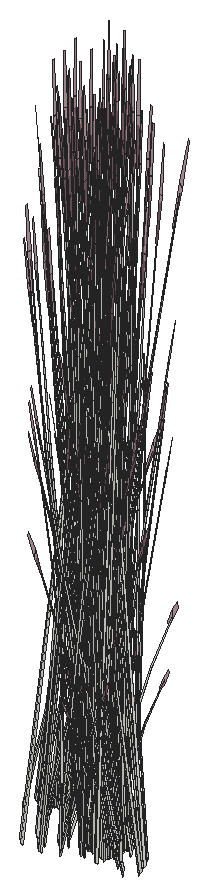
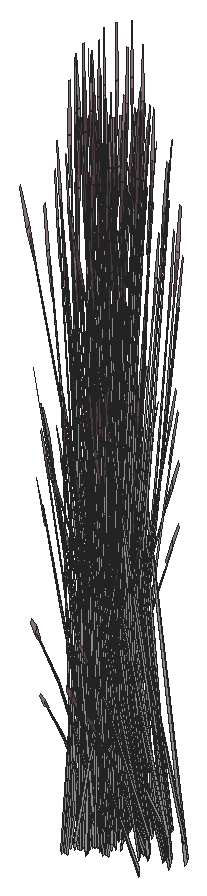
# SketchUp Ruby script. Lengths in inches.
U = 1.inch
M = Sketchup.active_model
def pt(a) = Geom::Point3d.new(a.map { |v| v * U })
def face(e, loops, mat)
  f = e.add_face(loops[0].map { |a| pt(a) })
  loops[1..].each { |l| e.add_face(l.map { |a| pt(a) }).erase! }
  f.material = f.back_material = mat if mat
  f
end
# faces: each face lists its corners as indices into pts; further lists are holes
def faces(e, pts, list, mat = nil) = list.each { |f| face(e, (f[0].is_a?(Array) ? f : [f]).map { |l| l.map { |i| pts[i] } }, mat) }
# xy, xz, yz: faces in a plane at the given z, y or x. An outline is a flat list of corners, or four numbers for a rectangle; further outlines are holes
def ring(l) = l.size == 4 ? [[l[0], l[1]], [l[2], l[1]], [l[2], l[3]], [l[0], l[3]]] : l.each_slice(2).to_a
def flat(e, list, mat, &to3) = list.each { |f| face(e, (f[0].is_a?(Array) ? f : [f]).map { |l| ring(l).map { |u, v| to3.(u, v) } }, mat) }
def xy(e, z, list, mat = nil) = flat(e, list, mat) { |x, y| [x, y, z] }
def xz(e, y, list, mat = nil) = flat(e, list, mat) { |x, z| [x, y, z] }
def yz(e, x, list, mat = nil) = flat(e, list, mat) { |y, z| [x, y, z] }
def lines(e, pts, list) = list.each { |a, b| e.add_line(pt(pts[a]), pt(pts[b])) }
# prism: a flat outline (further loops are holes) pulled along v
def prism(e, loops, v, mat = nil)
  f = face(e, loops, mat); d = Geom::Vector3d.new(v.map { |x| x * U })
  f.pushpull(f.normal.samedirection?(d) ? d.length : -d.length)
end
def box(e, o, s, mat = nil) = prism(e, [[o, [o[0] + s[0], o[1], o[2]], [o[0] + s[0], o[1] + s[1], o[2]], [o[0], o[1] + s[1], o[2]]]], [0, 0, s[2]], mat)
def at(x, y, z, deg = 0) = Geom::Transformation.translation(pt([x, y, z])) * Geom::Transformation.rotation(ORIGIN, Z_AXIS, deg.degrees)
def axes(o, x, y, z) = Geom::Transformation.new([*x, 0, *y, 0, *z, 0, *pt(o).to_a, 1])
def part(name) = M.definitions.add(name)
# library, detail: a bought-in or finely detailed component or shape, given as its bounding box
def library(name, o, s) = part(name).tap { |d| box(d.entities, o, s) }
def detail(e, o, s) = box(e.add_group.entities, o, s)
def put(e, d, t, mat = nil) = e.add_instance(d, t).tap { |i| i.material = mat if mat }
def group(e, t, mat = nil) = e.add_group.tap { |g| g.transformation = t; g.material = mat if mat }.entities
root = M.entities
M.materials.add("LightPink_Translucent").color = [144, 107, 117]
M.materials["LightPink_Translucent"].alpha = 0.75
c1 = part("blade")
p = [[2.15,0.21,22],[0,0.17,0],[0.09,0.45,0],[2.18,0.31,22],[2.29,0.31,22],[0.38,0.45,0],
  [2.48,0.24,33],[2.49,0.24,33],[2.48,0.22,33]]
faces(c1.entities,p,[[0,1,2,3],[4,5,2,3],[6,3,4,7],[8,0,3,6]])
c2 = part("seeds")
p = [[0.3,-0.1,1.38],[-0.01,-0.03,1.59],[-0.01,-0.03,0.03],[0.14,-0.07,-0.07],[0.29,-0.03,3],[0.15,0.01,3.11]]
faces(c2.entities,p,[[0,1,2,3],[1,0,4,5]],"LightPink_Translucent")
c3 = part("blade with seeds")
put(c3.entities,c1,at(0,0,0))
put(c3.entities,c2,axes([2.4,0.25,30.99],[1.5799,-0.05474,1.17369],[-0.12525,1.92788,0.29478],[-0.07173,-0.02425,1.56792]))
put(root,c3,axes([348.41,652.44,624.42],[-0.08753,-0.42921,0.48003],[0.34336,-0.07449,0.3958],[-0.1012,0.10094,0.9933]))
put(root,c3,axes([344.4,651.66,624.44],[-0.09971,0.42522,0.48003],[-0.32782,-0.1454,0.3958],[0.12892,-0.02555,0.9933]))
put(root,c3,axes([348.7,652.1,622.89],[-0.35635,0.30962,-0.29095],[-0.23697,-0.43749,-0.50002],[-0.08792,-0.04443,1.59708]))
put(root,c3,axes([347.72,653.07,624.96],[-0.25132,-0.3182,0.48003],[0.2669,-0.27442,0.3958],[-0.04636,0.14929,0.9933]))
put(root,c3,axes([348.34,652.36,624.42],[-0.2423,-0.19613,0.0643],[0.14107,-0.2793,0.50621],[-0.07768,0.0903,0.77189]))
put(root,c3,axes([345.14,652.99,624.78],[-0.05451,-0.37564,0.35414],[0.31161,-0.09919,-0.4572],[0.0837,0.10765,0.87481]))
put(root,c3,axes([347.9,652.75,622.25],[-0.08291,-0.40636,-0.30978],[0.32928,-0.11539,0.30978],[-0.06638,-0.04686,1.38974]))
put(root,c3,axes([347.625,653.04,624.96],[-0.29004,-0.02173,0.0643],[0.00795,-0.32812,0.50621],[-0.03035,0.12569,0.77189]))
put(root,c3,axes([345.21,651.02,621.9375],[0.21202,0.39143,-0.44739],[-0.32115,0.27564,0.21531],[0.06861,0.04843,1.43643]))
put(root,c3,axes([345.35,650.82,624.2],[-0.30498,-0.24231,1.38283],[0.32203,-0.37727,0.59665],[0.0984,0.22736,1.33663]))
put(root,c3,axes([344.19,652.38,624.42],[0.07571,-0.00789,1.74944],[0.20767,-0.36231,-0.27667],[0.13467,0.04783,0.14031]))
put(root,c3,axes([344.84,653.51,624.43],[0.00104,-0.05646,1.77383],[0.30246,-0.2491,-0.16761],[0.10506,0.08891,0.31391]))
put(root,c3,axes([348.9375,652.43,622.28],[-0.23773,0.35053,-0.62353],[-0.29532,-0.31785,-0.16365],[-0.09526,0.08744,1.37633]))
put(root,c3,axes([345.8125,652.8,622.49],[-0.19872,-0.13409,1.1486],[0.2566,-0.13625,0.84392],[0.06921,0.11541,0.25299]))
put(root,c3,axes([348.57,651.39,624.74],[0.29332,0.1301,0.35414],[-0.08555,0.37955,-0.4572],[-0.11809,0.0348,0.87481]))
put(root,c3,axes([345.09,651.7,622.47],[-0.21807,0.07699,1.1486],[0.10265,-0.31819,0.84392],[0.11568,0.02177,0.25299]))
put(root,c3,axes([348.625,652.57,624.37],[0.09067,0.42583,-0.51099],[-0.34336,0.07449,-0.3958],[-0.0984,0.11438,0.97773]))
put(root,c3,axes([349.48,652.26,621.75],[-0.36714,-0.07646,-0.62353],[0.07747,-0.47163,-0.16365],[-0.10956,-0.05715,1.37633]))
put(root,c3,axes([349.1,652.24,622.69],[-0.34464,-0.37536,-0.25192],[0.29,-0.42149,0.5513],[-0.0928,0.04391,1.68216]))
put(root,c3,axes([348.48,651.875,622.4375],[-0.21202,-0.39143,-0.44739],[0.32115,-0.27564,0.21531],[-0.06861,-0.04843,1.43643]))
put(root,c3,axes([344.47,651.62,624.23],[0.29332,0.1301,-0.35414],[-0.08555,0.37955,0.4572],[0.11809,-0.0348,0.87481]))
put(root,c3,axes([348.9,650.57,624.74],[0.20082,0.29199,0.35414],[-0.2293,0.2764,-0.4572],[-0.1165,-0.04206,0.87481]))
put(root,c3,axes([345.79,650.15,621.75],[0.08291,0.40636,-0.30978],[-0.32928,0.11539,0.30978],[0.06638,0.04686,1.38974]))
put(root,c3,axes([346.41,651.48,622.1],[0.44133,0,0],[0,0.52122,-0.51607],[0,0.11871,1.63711]))
put(root,c3,axes([343.9,652.4375,624.6875],[0.35281,0.01123,-0.71045],[-0.0237,0.47284,0.08574],[0.14947,0.0499,1.00501]))
put(root,c3,axes([348.93,652.16,622.4375],[-0.38326,0.02879,-0.44739],[-0.03466,-0.47788,0.21531],[-0.06861,0.04843,1.43643]))
put(root,c3,axes([344.98,650.8,622.39],[0.35635,-0.30962,-0.29095],[0.23697,0.43749,-0.50002],[0.08792,0.04443,1.59708]))
put(root,c3,axes([344.62,651.54,621.69],[-0.22732,0.05597,1.41583],[-0.03618,-0.44548,0.08104],[0.15921,-0.06743,0.80566]))
put(root,c3,axes([345.84,653.41,622.39],[-0.22633,-0.01463,1.0506],[0.14947,-0.31064,0.58006],[0.08941,0.11036,0.8241]))
put(root,c3,axes([349,653.16,621.71],[-0.33032,-0.23318,-0.49651],[0.19744,-0.41812,0],[-0.07523,-0.05311,1.57504]))
put(root,c3,axes([344.87,651.25,621.2],[-0.01845,-0.0708,1.76342],[0.12793,-0.41416,-0.26939],[0.12905,-0.00596,0.30037]))
put(root,c3,axes([348.46,652.26,624.73],[0.32648,0.25715,-0.1216],[-0.18809,0.3724,-0.67495],[-0.09224,0.12945,1.02557]))
put(root,c3,axes([344.99,653.04,624.42],[-0.03191,-0.04083,1.77383],[0.06981,-0.43764,-0.16761],[0.12571,-0.02796,0.31391]))
put(root,c3,axes([343.67,651.15,623.58],[-0.14639,0.01056,1.71376],[0.09712,-0.45778,0.13857],[0.20862,0.02831,0.73262]))
put(root,c3,axes([348.2,652.96,622.7],[0.33032,0.23318,0.49651],[-0.19744,0.41812,0],[-0.07523,-0.05311,1.57504]))
put(root,c3,axes([349.2,653.4375,622.0625],[-0.22066,0.46731,0],[-0.36918,-0.26061,-0.51607],[-0.08408,-0.05936,1.63711]))
put(root,c3,axes([345.11,653.18,624.76],[0.21031,-0.39918,-0.1216],[0.30457,0.22997,-0.67495],[0.10587,0.11278,1.02557]))
put(root,c3,axes([344.2,651.58,624.6875],[0.31014,-0.20596,-0.71045],[0.17284,0.42397,0.08574],[0.14985,-0.04816,1.00501]))
put(root,c3,axes([348.67,652.23,622.84],[-0.06809,0.4162,0.1448],[-0.33266,-0.07225,-0.41347],[-0.06054,-0.04274,1.26744]))
put(root,c3,axes([344.08,650.53,621.32],[-0.3474,0.18671,1.28929],[-0.11057,-0.53572,0.50096],[0.21332,0.00891,1.46642]))
put(root,c3,axes([347.92,653.38,625.34],[0.31145,0.12449,-0.06488],[-0.0958,0.38314,-0.29416],[-0.05094,0.05817,0.97024]))
put(root,c3,axes([349.33,653.39,622.24],[-0.33032,0.23318,-0.49651],[-0.19744,-0.41812,0],[-0.07523,0.05311,1.57504]))
put(root,c3,axes([349.35,653.27,622.42],[-0.21791,-0.46895,-0.05142],[0.36918,-0.26061,0.51607],[-0.09097,0.04465,1.6363]))
put(root,c3,axes([348.62,652.3,624.74],[0.30722,-0.06665,0.35414],[0.08112,0.381,-0.4572],[-0.08804,0.10234,0.87481]))
put(root,c3,axes([345.36,652.98,624.41],[0.34827,-0.11086,-0.51099],[0.06092,0.41983,-0.3958],[0.09354,0.12031,0.97773]))
put(root,c3,axes([349.25,653.21,622.25],[-0.32928,-0.11539,-0.30978],[0.08291,-0.40636,0.30978],[-0.06638,0.04686,1.38974]))
put(root,c3,axes([347.84,652.82,625.28],[0.23881,-0.24554,0.35414],[0.22606,0.28036,-0.4572],[-0.0344,0.14245,0.87481]))
put(root,c3,axes([345.76,652.48,624.78],[-0.20082,-0.29199,0.35414],[0.2293,-0.2764,-0.4572],[0.1165,0.04206,0.87481]))
put(root,c3,axes([349.44,651.47,623.07],[-0.00964,-0.43909,1.41272],[0.43635,0.11382,0.59816],[-0.1032,0.24027,1.3335]))
put(root,c3,axes([345.88,649.98,621.74],[0.33032,0.23318,-0.49651],[-0.19744,0.41812,0],[0.07523,0.05311,1.57504]))
put(root,c3,axes([344.68,652.21,622.3],[-0.085,-0.1147,1.43002],[0.1106,-0.37943,-0.30754],[0.17198,0.0514,0.61141]))
put(root,c3,axes([345.94,652.74,624.46],[-0.01777,0.35463,0.0643],[-0.26836,-0.00972,0.50621],[0.1028,0.03711,0.77189]))
put(root,c3,axes([349.9,652.33,622.36],[-0.35635,0.30962,-0.29095],[-0.23697,-0.43749,-0.50002],[-0.08792,-0.04443,1.59708]))
put(root,c3,axes([345.87,653.3,621.22],[0.02571,-0.06733,1.76342],[0.32373,-0.19829,-0.26939],[0.09815,0.10263,0.30037]))
put(root,c3,axes([345.97,652.63,624.46],[-0.26024,0.30729,0.48003],[-0.22444,-0.32634,0.3958],[0.1221,0.05668,0.9933]))
put(root,c3,axes([348.91,653.3125,624.42],[-0.25132,-0.3182,0.48003],[0.2669,-0.27442,0.3958],[-0.04636,0.14929,0.9933]))
put(root,c3,axes([349.2,652.03,622.89],[0.04113,0.53214,-0.29095],[-0.42835,0.03218,-0.50002],[-0.07543,0.07088,1.59708]))
put(root,c3,axes([346.64,652.68,623.66],[-0.06755,-0.39203,-0.03492],[0.31928,-0.09013,-0.15832],[0.06667,0.02485,0.52218]))
put(root,c3,axes([351.41,651.85,623.01],[0.14639,-0.01056,1.71376],[-0.09712,0.45778,0.13857],[-0.20862,-0.02831,0.73262]))
put(root,c3,axes([346.09,651.66,624.78],[-0.29332,-0.1301,0.35414],[0.08555,-0.37955,-0.4572],[0.11809,-0.0348,0.87481]))
put(root,c3,axes([349.09,652.98,621.72],[-0.08291,-0.40636,-0.30978],[0.32928,-0.11539,0.30978],[-0.06638,-0.04686,1.38974]))
put(root,c3,axes([348.82,653.28,624.42],[-0.29004,-0.02173,0.0643],[0.00795,-0.32812,0.50621],[-0.03035,0.12569,0.77189]))
put(root,c3,axes([345.4,650.87,621.78],[0.36714,0.07646,-0.62353],[-0.07747,0.47163,-0.16365],[0.10956,0.05715,1.37633]))
put(root,c3,axes([346.96,651.15,621.99],[-0.21881,-0.29821,-0.06488],[0.23965,-0.27324,-0.29416],[0.0679,-0.01924,0.97024]))
put(root,c3,axes([348.56,651.83,622.59],[0.44609,0.09826,0.45755],[-0.09078,0.55493,0.17955],[-0.06519,-0.05359,1.58856]))
put(root,c3,axes([350.13,652.67,621.75],[-0.23773,0.35053,-0.62353],[-0.29532,-0.31785,-0.16365],[-0.09526,0.08744,1.37633]))
put(root,c3,axes([348.44,651.73,622.94],[-0.17124,0.42022,0.44739],[-0.35581,-0.20224,-0.21531],[0,-0.09687,1.43643]))
put(root,c3,axes([350.3,652.47,622.16],[-0.34464,-0.37536,-0.25192],[0.29,-0.42149,0.5513],[-0.0928,0.04391,1.68216]))
put(root,c3,axes([351.47,652.66,623.01],[0.12246,-0.09864,1.71376],[0.1031,0.45582,0.13857],[-0.19225,0.10302,0.73262]))
put(root,c3,axes([349.67,652.11,621.9],[-0.21202,-0.39143,-0.44739],[0.32115,-0.27564,0.21531],[-0.06861,-0.04843,1.43643]))
put(root,c3,axes([345.33,651.88,623.6],[-0.1311,-0.08035,1.71376],[0.27131,-0.33708,0.13857],[0.16909,0.15206,0.73262]))
put(root,c3,axes([351.09,653.43,621.73],[0.12266,0.03828,1.43002],[0.07906,0.39104,-0.30754],[-0.16661,0.0732,0.61141]))
put(root,c3,axes([348.32,652.72,622.7],[0.37926,-0.12378,0.17642],[0.09365,0.46065,0.35086],[-0.03382,-0.06712,1.60407]))
put(root,c3,axes([350.12,652.39,621.9],[-0.38326,0.02879,-0.44739],[-0.03466,-0.47788,0.21531],[-0.06861,0.04843,1.43643]))
put(root,c3,axes([348.81,652.79,622.42],[-0.35581,-0.20937,0],[0.17124,-0.43505,0],[0,0,1.62707]))
put(root,c3,axes([349.63,653.32,622.6],[0.22066,0.46731,0],[-0.36918,0.26061,-0.51607],[-0.08408,0.05936,1.63711]))
put(root,c3,axes([346.36,651.78,624.46],[0.12963,0.31798,0.0643],[-0.23638,0.15564,0.50621],[0.1042,-0.03071,0.77189]))
put(root,c3,axes([352.17,652.18,622.48],[0.10032,-0.06746,1.77064],[0.0346,0.47103,0.13857],[-0.2173,0.0625,0.63284]))
put(root,c3,axes([346.05,652.63,624.25],[0.20082,0.29199,-0.35414],[-0.2293,0.2764,0.4572],[0.1165,0.04206,0.87481]))
put(root,c3,axes([345.82,652.66,624.76],[0.0189,-0.47427,-0.1216],[0.35781,0.01296,-0.67495],[0.13781,0.03295,1.02557]))
put(root,c3,axes([346.33,651.66,624.46],[-0.09971,0.42522,0.48003],[-0.32782,-0.1454,0.3958],[0.12892,-0.02555,0.9933]))
put(root,c3,axes([349.39,653.19,622.17],[0.33032,0.23318,0.49651],[-0.19744,0.41812,0],[-0.07523,-0.05311,1.57504]))
put(root,c3,axes([349.45,652.75,622.7],[0.10196,-0.46348,0.17642],[0.3731,0.13116,0.35086],[-0.06445,0.00226,1.60407]))
put(root,c3,axes([349.28,652.13,622.84],[0.26075,0.2802,0.1448],[-0.2175,0.31612,-0.41347],[-0.06054,0.04274,1.26744]))
put(root,c3,axes([349.18,651.79,622.52],[-0.32829,-0.4014,-0.06131],[0.32849,-0.40164,0],[-0.01146,-0.01402,1.75571]))
put(root,c3,axes([349.27,651.93,622.94],[0.38326,-0.02879,0.44739],[0.03466,0.47788,-0.21531],[-0.06861,0.04843,1.43643]))
put(root,c3,axes([349.86,652.47,622.31],[-0.06809,0.4162,0.1448],[-0.33266,-0.07225,-0.41347],[-0.06054,-0.04274,1.26744]))
put(root,c3,axes([351.09,652.5,623.85],[-0.05763,0.06055,1.74944],[0.0049,0.44239,-0.27667],[-0.13211,0.05753,0.14031]))
put(root,c3,axes([351.85,651.42,624.12],[-0.35281,-0.01123,-0.71045],[0.0237,-0.47284,0.08574],[-0.14947,-0.0499,1.00501]))
put(root,c3,axes([350.52,653.63,621.71],[-0.33032,0.23318,-0.49651],[-0.19744,-0.41812,0],[-0.07523,0.05311,1.57504]))
put(root,c3,axes([349.36,653.02,622.56],[0.44186,0.15158,0.30756],[-0.11054,0.54181,-0.36492],[-0.07313,0.06781,1.64885]))
put(root,c3,axes([348.74,651.74,622.17],[0,0.46636,0.49651],[-0.39487,0,0],[0,-0.10622,1.57504]))
put(root,c3,axes([350.55,653.5,621.88],[-0.21791,-0.46895,-0.05142],[0.36918,-0.26061,0.51607],[-0.09097,0.04465,1.6363]))
put(root,c3,axes([351.5625,651.54,621.73],[0.06891,0.12984,1.43002],[-0.15879,0.35293,-0.30754],[-0.16304,-0.08436,0.61141]))
put(root,c3,axes([349.55,652.99,622.7],[0.33032,-0.23318,0.49651],[0.19744,0.41812,0],[-0.07523,0.05311,1.57504]))
put(root,c3,axes([346.13,652.38,624.44],[0.07571,-0.00789,1.74944],[0.20767,-0.36231,-0.27667],[0.13467,0.04783,0.14031]))
put(root,c3,axes([351.28,652.24,623.66],[-0.29332,-0.1301,-0.35414],[0.08555,-0.37955,0.4572],[-0.11809,0.0348,0.87481]))
put(root,c3,axes([348.52,651.32,622.59],[0.15345,0.52148,0.45755],[-0.43845,0.18134,0.17955],[0.00536,-0.09582,1.58856]))
put(root,c3,axes([350.45,653.44,621.72],[-0.32928,-0.11539,-0.30978],[0.08291,-0.40636,0.30978],[-0.06638,0.04686,1.38974]))
put(root,c3,axes([348.89,652.61,622.43],[-0.11516,-0.40207,0],[0.32884,-0.1408,0],[0,0,1.54371]))
put(root,c3,axes([349.04,653.06,624.74],[0.23881,-0.24554,0.35414],[0.22606,0.28036,-0.4572],[-0.0344,0.14245,0.87481]))
put(root,c3,axes([347.02,651.7,622.49],[-0.21807,0.07699,1.1486],[0.10265,-0.31819,0.84392],[0.11568,0.02177,0.25299]))
put(root,c3,axes([350.64,651.71,622.53],[-0.00964,-0.43909,1.41272],[0.43635,0.11382,0.59816],[-0.1032,0.24027,1.3335]))
put(root,c3,axes([350.45,652.94,623.85],[0.04504,0.01251,1.77383],[0.13934,0.41205,-0.16761],[-0.0922,0.10815,0.31391]))
put(root,c3,axes([351.48,652.4375,623.82],[-0.09562,0.42421,-0.51099],[-0.32782,-0.1454,-0.3958],[-0.13199,0.0389,0.97773]))
put(root,c3,axes([346.4,651.62,624.25],[0.29332,0.1301,-0.35414],[-0.08555,0.37955,0.4572],[0.11809,-0.0348,0.87481]))
put(root,c3,axes([351.73,651.52,623.82],[-0.25628,0.30892,-0.51099],[-0.22444,-0.32634,-0.3958],[-0.13021,-0.047,0.97773]))
put(root,c3,axes([351.32,652.41,620.63],[0.00895,0.0735,1.76342],[-0.18044,0.38382,-0.26939],[-0.12817,-0.01935,0.30037]))
put(root,c3,axes([350.39,652.27,622.36],[0.04113,0.53214,-0.29095],[-0.42835,0.03218,-0.50002],[-0.07543,0.07088,1.59708]))
put(root,c3,axes([349.35,651.82,622.4375],[-0.17124,0.42022,-0.44739],[-0.35581,-0.20224,0.21531],[0,0.09687,1.43643]))
put(root,c3,axes([345.83,652.4375,624.71],[0.35281,0.01123,-0.71045],[-0.0237,0.47284,0.08574],[0.14947,0.0499,1.00501]))
put(root,c3,axes([351.37,650.65,623.85],[0.02617,0.04654,1.77383],[-0.12614,0.41836,-0.16761],[-0.12775,0.00303,0.31391]))
put(root,c3,axes([346.55,651.54,621.71],[-0.22732,0.05597,1.41583],[-0.03618,-0.44548,0.08104],[0.15921,-0.06743,0.80566]))
put(root,c3,axes([350.83,654.25,621.9],[0.14709,-0.21136,1.1486],[0.05804,0.3346,0.84392],[-0.1063,0.05991,0.25299]))
put(root,c3,axes([350.03,651.5625,622.7],[-0.2773,-0.3397,0.17642],[0.27945,-0.32949,0.35086],[-0.03063,0.06937,1.60407]))
put(root,c3,axes([346.8,651.25,621.22],[-0.01845,-0.0708,1.76342],[0.12793,-0.41416,-0.26939],[0.12905,-0.00596,0.30037]))
put(root,c3,axes([349.07,651.37,622.43],[0,-0.53961,0],[0.44133,0,0],[0,0,1.79456]))
put(root,c3,axes([346.92,653.04,624.43],[-0.03191,-0.04083,1.77383],[0.06981,-0.43764,-0.16761],[0.12571,-0.02796,0.31391]))
put(root,c3,axes([345.6,651.15,623.6],[-0.14639,0.01056,1.71376],[0.09712,-0.45778,0.13857],[0.20862,0.02831,0.73262]))
put(root,c3,axes([349.75,652.07,622.05],[0.44609,0.09826,0.45755],[-0.09078,0.55493,0.17955],[-0.06519,-0.05359,1.58856]))
put(root,c3,axes([349.29,651.58,622.52],[0,0.53934,-0.05637],[-0.44133,0,0],[0,0.01695,1.79368]))
put(root,c3,axes([351.35,652.2,623.87],[0.09971,-0.42522,0.48003],[0.32782,0.1454,0.3958],[-0.12892,0.02555,0.9933]))
put(root,c3,axes([348.51,653.23,625.28],[0.1064,-0.35863,0.35414],[0.31043,0.1046,-0.4572],[0.02846,0.14439,0.87481]))
put(root,c3,axes([351.46,652.07,624.17],[0.17758,0.42229,-0.1216],[-0.31518,0.20752,-0.67495],[-0.13282,0.05572,1.02557]))
put(root,c3,axes([351.86,651.2,624.17],[-0.0189,0.47427,-0.1216],[-0.35781,-0.01296,-0.67495],[-0.13781,-0.03295,1.02557]))
put(root,c3,axes([351.32,652.08,623.87],[-0.12963,-0.31798,0.0643],[0.23638,-0.15564,0.50621],[-0.1042,0.03071,0.77189]))
put(root,c3,axes([348.35,650.33,622.7],[-0.10196,0.46348,0.17642],[-0.3731,-0.13116,0.35086],[0.06445,-0.00226,1.60407]))
put(root,c3,axes([349.08,652.625,622.52],[0.15345,0.53576,-0.06012],[-0.43845,0.18773,0],[0.00536,0.01871,1.72173]))
put(root,c3,axes([349.64,651.97,622.41],[-0.17124,0.42022,0.44739],[-0.35581,-0.20224,-0.21531],[0,-0.09687,1.43643]))
put(root,c3,axes([351.39,653.34,623.66],[-0.30722,0.06665,-0.35414],[-0.08112,-0.381,0.4572],[-0.08804,0.10234,0.87481]))
put(root,c3,axes([346.14,651.58,624.71],[0.31014,-0.20596,-0.71045],[0.17284,0.42397,0.08574],[0.14985,-0.04816,1.00501]))
put(root,c3,axes([351.15,651.93,621.9],[0.22533,-0.03337,1.1486],[-0.14293,0.29403,0.84392],[-0.11135,-0.04411,0.25299]))
put(root,c3,axes([350.35,651.92,622.42],[-0.44111,-0.00373,-0.04976],[0,-0.52122,0.49943],[-0.01386,0.11865,1.58352]))
put(root,c3,axes([349.51,652.96,622.16],[0.37926,-0.12378,0.17642],[0.09365,0.46065,0.35086],[-0.03382,-0.06712,1.60407]))
put(root,c3,axes([350,653.03,621.89],[-0.35581,-0.20937,0],[0.17124,-0.43505,0],[0,0,1.62707]))
put(root,c3,axes([349.48,650.36,622.7],[-0.37926,0.12378,0.17642],[-0.09365,-0.46065,0.35086],[0.03382,0.06712,1.60407]))
put(root,c3,axes([351.43,653.26,623.87],[-0.08753,-0.42921,0.48003],[0.34336,-0.07449,0.3958],[-0.1012,0.10094,0.9933]))
put(root,c3,axes([350.82,653.56,622.0625],[0.22066,0.46731,0],[-0.36918,0.26061,-0.51607],[-0.08408,0.05936,1.63711]))
put(root,c3,axes([348.93,654.5,625.87],[0.2439,-0.26754,-0.06488],[0.22348,0.29302,-0.29416],[0.01573,0.08303,0.97024]))
put(root,c3,axes([346.61,652.21,622.32],[-0.085,-0.1147,1.43002],[0.1106,-0.37943,-0.30754],[0.17198,0.0514,0.61141]))
put(root,c3,axes([351.36,653.17,623.87],[-0.2423,-0.19613,0.0643],[0.14107,-0.2793,0.50621],[-0.07768,0.0903,0.77189]))
put(root,c3,axes([348.86,651.03,622.59],[-0.29264,0.42323,0.45755],[-0.34767,-0.3736,0.17955],[0.07055,-0.04224,1.58856]))
put(root,c3,axes([349.36,651.7,622.4375],[0.24637,0.30123,0],[-0.24637,0.30123,0],[0,0,1.69266]))
put(root,c3,axes([349.36,651.34,622.94],[0.17124,-0.42022,0.44739],[0.35581,0.20224,-0.21531],[0,0.09687,1.43643]))
put(root,c3,axes([349.21,652.8,622.43],[0.35581,0.20937,0],[-0.17124,0.43505,0],[0,0,1.74954]))
put(root,c3,axes([350.64,652.98,622.16],[0.10196,-0.46348,0.17642],[0.3731,0.13116,0.35086],[-0.06445,0.00226,1.60407]))
put(root,c3,axes([350.47,652.37,622.31],[0.26075,0.2802,0.1448],[-0.2175,0.31612,-0.41347],[-0.06054,0.04274,1.26744]))
put(root,c3,axes([350.375,652.02,621.99],[-0.32829,-0.4014,-0.06131],[0.32849,-0.40164,0],[-0.01146,-0.01402,1.75571]))
put(root,c3,axes([350.46,652.16,622.41],[0.38326,-0.02879,0.44739],[0.03466,0.47788,-0.21531],[-0.06861,0.04843,1.43643]))
put(root,c3,axes([349.24,651.24,622.61],[-0.44609,-0.09826,0.49198],[0.09078,-0.55493,0.19306],[0.06519,0.05359,1.70813]))
put(root,c3,axes([350.56,653.26,622.02],[0.44186,0.15158,0.30756],[-0.11054,0.54181,-0.36492],[-0.07313,0.06781,1.64885]))
put(root,c3,axes([350.26,652,622.25],[-0.24637,0.29097,-0.30978],[-0.24637,-0.29097,0.30978],[0,0.09372,1.38974]))
put(root,c3,axes([351.59,652.2,624.1875],[0.29332,0.1301,0.35414],[-0.08555,0.37955,-0.4572],[-0.11809,0.0348,0.87481]))
put(root,c3,axes([350.75,653.23,622.17],[0.33032,-0.23318,0.49651],[0.19744,0.41812,0],[-0.07523,0.05311,1.57504]))
put(root,c3,axes([349.55,651.95,622.32],[0.12941,0.42699,-0.69212],[-0.37279,0.15378,-0.18165],[0.0143,0.14459,1.52773]))
put(root,c3,axes([349.37,651.49,622.43],[0.39487,0,0],[0,0.48281,0],[0,0,1.78407]))
put(root,c3,axes([349.71,651.5625,622.05],[0.15345,0.52148,0.45755],[-0.43845,0.18134,0.17955],[0.00536,-0.09582,1.58856]))
put(root,c3,axes([350.08,652.85,621.89],[-0.11516,-0.40207,0],[0.32884,-0.1408,0],[0,0,1.54371]))
put(root,c3,axes([348.99,650.96,622.94],[-0.21202,-0.39143,0.44739],[0.32115,-0.27564,-0.21531],[0.06861,0.04843,1.43643]))
put(root,c3,axes([352.5,653.08,621.2],[-0.36714,-0.07646,-0.62353],[0.07747,-0.47163,-0.16365],[-0.10956,-0.05715,1.37633]))
put(root,c3,axes([349.51,651.4375,622.84],[0.32884,-0.136,0.1448],[0.11516,0.38837,-0.41347],[0,0.08547,1.26744]))
put(root,c3,axes([351.92,651.38,624.1875],[0.20082,0.29199,0.35414],[-0.2293,0.2764,-0.4572],[-0.1165,-0.04206,0.87481]))
put(root,c3,axes([349.4,651.47,622.89],[0.39748,0.22252,-0.29095],[-0.19139,0.46966,-0.50002],[0.01249,0.11531,1.59708]))
put(root,c3,axes([352.01,653.97,621.16],[-0.33032,-0.23318,-0.49651],[0.19744,-0.41812,0],[-0.07523,-0.05311,1.57504]))
put(root,c3,axes([350.55,652.06,621.9],[-0.17124,0.42022,-0.44739],[-0.35581,-0.20224,0.21531],[0,0.09687,1.43643]))
put(root,c3,axes([352.21,654.25,621.51],[-0.22066,0.46731,0],[-0.36918,-0.26061,-0.51607],[-0.08408,-0.05936,1.63711]))
put(root,c3,axes([351.22,651.8,622.16],[-0.2773,-0.3397,0.17642],[0.27945,-0.32949,0.35086],[-0.03063,0.06937,1.60407]))
put(root,c3,axes([350.26,651.58,622.7],[0,-0.46636,0.49651],[0.39487,0,0],[0,0.10622,1.57504]))
put(root,c3,axes([350.43,652.01,622.24],[0,0.46636,-0.49651],[-0.39487,0,0],[0,0.10622,1.57504]))
put(root,c3,axes([349.375,653.42,624.96],[-0.35104,0.10702,0.48003],[-0.06092,-0.41983,0.3958],[0.08256,0.12373,0.9933]))
put(root,c3,axes([350.27,651.61,621.9],[0,-0.53961,0],[0.44133,0,0],[0,0,1.79456]))
put(root,c3,axes([349.31,653.51,624.96],[-0.16041,0.29625,0.0643],[-0.22843,-0.17248,0.50621],[0.07385,0.09498,0.77189]))
put(root,c3,axes([350.49,651.82,621.98],[0,0.53934,-0.05637],[-0.44133,0,0],[0,0.01695,1.79368]))
put(root,c3,axes([349.13,650.85,622.84],[0.06809,-0.4162,0.1448],[0.33266,0.07225,-0.41347],[0.06054,0.04274,1.26744]))
put(root,c3,axes([349.73,651.39,622.41],[-0.38326,0.02879,0.44739],[-0.03466,-0.47788,-0.21531],[0.06861,-0.04843,1.43643]))
put(root,c3,axes([349.7,653.46,624.74],[0.1064,-0.35863,0.35414],[0.31043,0.1046,-0.4572],[0.02846,0.14439,0.87481]))
put(root,c3,axes([350.9375,654.19,624.78],[0.31145,0.12449,-0.06488],[-0.0958,0.38314,-0.29416],[-0.05094,0.05817,0.97024]))
put(root,c3,axes([349.55,650.57,622.16],[-0.10196,0.46348,0.17642],[-0.3731,-0.13116,0.35086],[0.06445,-0.00226,1.60407]))
put(root,c3,axes([351.64,653.11,624.1875],[0.30722,-0.06665,0.35414],[0.08112,0.381,-0.4572],[-0.08804,0.10234,0.87481]))
put(root,c3,axes([350.28,652.86,621.98],[0.15345,0.53576,-0.06012],[-0.43845,0.18773,0],[0.00536,0.01871,1.72173]))
put(root,c3,axes([349.61,650.12,622.7],[-0.33032,-0.23318,0.49651],[0.19744,-0.41812,0],[0.07523,0.05311,1.57504]))
put(root,c3,axes([349.32,652.56,622.41],[0.37054,-0.15823,-0.19198],[0.1302,0.45581,0.00008],[0.0409,-0.01749,1.73897]))
put(root,c3,axes([351.54,652.16,621.89],[-0.44111,-0.00373,-0.04976],[0,-0.52122,0.49943],[-0.01386,0.11865,1.58352]))
put(root,c3,axes([350.68,650.59,622.16],[-0.37926,0.12378,0.17642],[-0.09365,-0.46065,0.35086],[0.03382,0.06712,1.60407]))
put(root,c3,axes([352.91,653.15,621.8],[-0.35635,0.30962,-0.29095],[-0.23697,-0.43749,-0.50002],[-0.08792,-0.04443,1.59708]))
put(root,c3,axes([349.26,653.17,625.28],[-0.05451,-0.37564,0.35414],[0.31161,-0.09919,-0.4572],[0.0837,0.10765,0.87481]))
put(root,c3,axes([349.33,651.2,622.4375],[0.21202,0.39143,-0.44739],[-0.32115,0.27564,0.21531],[0.06861,0.04843,1.43643]))
put(root,c3,axes([350.06,651.27,622.05],[-0.29264,0.42323,0.45755],[-0.34767,-0.3736,0.17955],[0.07055,-0.04224,1.58856]))
put(root,c3,axes([352.11,653.8,621.17],[-0.08291,-0.40636,-0.30978],[0.32928,-0.11539,0.30978],[-0.06638,-0.04686,1.38974]))
put(root,c3,axes([350.56,651.93,621.91],[0.24637,0.30123,0],[-0.24637,0.30123,0],[0,0,1.69266]))
put(root,c3,axes([350.55,651.58,622.41],[0.17124,-0.42022,0.44739],[0.35581,0.20224,-0.21531],[0,0.09687,1.43643]))
put(root,c3,axes([349.47,651,624.7],[-0.30498,-0.24231,1.38283],[0.32203,-0.37727,0.59665],[0.0984,0.22736,1.33663]))
put(root,c3,axes([350.4,653.04,621.89],[0.35581,0.20937,0],[-0.17124,0.43505,0],[0,0,1.74954]))
put(root,c3,axes([348.95,653.69,624.93],[0.00104,-0.05646,1.77383],[0.30246,-0.2491,-0.16761],[0.10506,0.08891,0.31391]))
put(root,c3,axes([349.93,652.98,622.99],[-0.19872,-0.13409,1.1486],[0.2566,-0.13625,0.84392],[0.06921,0.11541,0.25299]))
put(root,c3,axes([350.4375,651.48,622.07],[-0.44609,-0.09826,0.49198],[0.09078,-0.55493,0.19306],[0.06519,0.05359,1.70813]))
